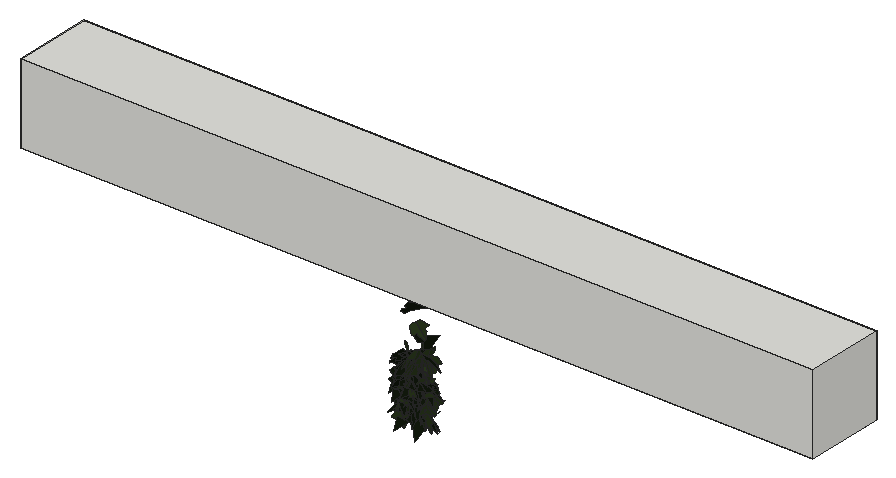
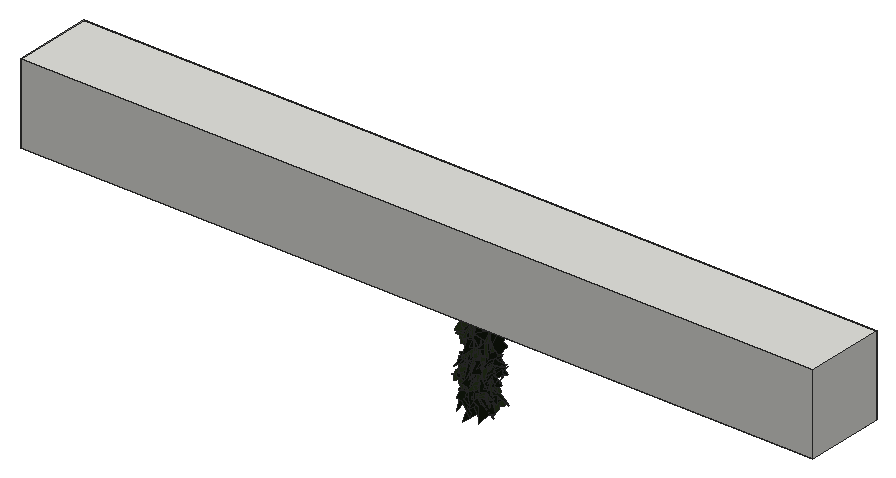
# SketchUp Ruby script. Lengths in inches.
U = 1.inch
M = Sketchup.active_model
def pt(a) = Geom::Point3d.new(a.map { |v| v * U })
def face(e, loops, mat)
  f = e.add_face(loops[0].map { |a| pt(a) })
  loops[1..].each { |l| e.add_face(l.map { |a| pt(a) }).erase! }
  f.material = f.back_material = mat if mat
  f
end
# faces: each face lists its corners as indices into pts; further lists are holes
def faces(e, pts, list, mat = nil) = list.each { |f| face(e, (f[0].is_a?(Array) ? f : [f]).map { |l| l.map { |i| pts[i] } }, mat) }
# xy, xz, yz: faces in a plane at the given z, y or x. An outline is a flat list of corners, or four numbers for a rectangle; further outlines are holes
def ring(l) = l.size == 4 ? [[l[0], l[1]], [l[2], l[1]], [l[2], l[3]], [l[0], l[3]]] : l.each_slice(2).to_a
def flat(e, list, mat, &to3) = list.each { |f| face(e, (f[0].is_a?(Array) ? f : [f]).map { |l| ring(l).map { |u, v| to3.(u, v) } }, mat) }
def xy(e, z, list, mat = nil) = flat(e, list, mat) { |x, y| [x, y, z] }
def xz(e, y, list, mat = nil) = flat(e, list, mat) { |x, z| [x, y, z] }
def yz(e, x, list, mat = nil) = flat(e, list, mat) { |y, z| [x, y, z] }
def lines(e, pts, list) = list.each { |a, b| e.add_line(pt(pts[a]), pt(pts[b])) }
# prism: a flat outline (further loops are holes) pulled along v
def prism(e, loops, v, mat = nil)
  f = face(e, loops, mat); d = Geom::Vector3d.new(v.map { |x| x * U })
  f.pushpull(f.normal.samedirection?(d) ? d.length : -d.length)
end
def box(e, o, s, mat = nil) = prism(e, [[o, [o[0] + s[0], o[1], o[2]], [o[0] + s[0], o[1] + s[1], o[2]], [o[0], o[1] + s[1], o[2]]]], [0, 0, s[2]], mat)
def at(x, y, z, deg = 0) = Geom::Transformation.translation(pt([x, y, z])) * Geom::Transformation.rotation(ORIGIN, Z_AXIS, deg.degrees)
def axes(o, x, y, z) = Geom::Transformation.new([*x, 0, *y, 0, *z, 0, *pt(o).to_a, 1])
def part(name) = M.definitions.add(name)
# library, detail: a bought-in or finely detailed component or shape, given as its bounding box
def library(name, o, s) = part(name).tap { |d| box(d.entities, o, s) }
def detail(e, o, s) = box(e.add_group.entities, o, s)
def put(e, d, t, mat = nil) = e.add_instance(d, t).tap { |i| i.material = mat if mat }
def group(e, t, mat = nil) = e.add_group.tap { |g| g.transformation = t; g.material = mat if mat }.entities
root = M.entities
M.materials.add("efeu1").color = [18, 25, 13]
M.materials.add("efeu2").color = [43, 57, 29]
c1 = part("ivyleaf_9")
p = [[1.54,2.16,1.25],[1.36,2.04,1.19],[-0.21,0.99,0.68],[-0.71,1.11,0.82],[-0.85,0.86,0.67],[-0.8,0.17,0.21],
  [-0.9,-0.01,0.1],[-0.67,-0.16,-0.02],[-0.08,-0.08,-0.05],[-0.03,-0.6,-0.4],[0.65,-0.88,-0.66],[0.83,-0.6,-0.49],
  [1.29,-0.42,-0.43],[1.8125,-0.07,-0.26],[1.21,0.44,0.15]]
faces(c1.entities,p,[[0,1,2,3,4,5,6,7,8,9,10,11,12,13,14]],"efeu1")
c2 = part("ivyleaf_10")
p = [[0,0.5,-0.03],[-0.0625,2.02,-0.43],[-0.19,2.01,-0.46],[-0.54,1.05,-0.29],[-0.52,0.625,-0.18],[-0.83,0.76,-0.28],
  [-1.16,0.64,-0.33],[-1.15,0.33,-0.24],[-0.77,-0.39,0.02],[-0.3,-0.51,0.16],[0.04,-0.48,0.23],[-0.02,2.01,-0.4375],
  [-0.06,2.01,-0.43],[0.04,-0.49,0.23],[0.67,-0.49,0.14],[1.38,0.36,-0.2],[1.375,0.51,-0.24],[0.81,0.65,-0.19],
  [0.62,0.59,-0.15],[0.6,1.09,-0.28],[0.5,1.23,-0.31]]
faces(c2.entities,p,[[0,1,2,3,4,5,6,7,8,9,10],[11,12,0,13,14,15,16,17,18,19,20]],"efeu2")
c3 = part("Agrupar\#1")
box(c3.entities,[0,0,0],[11.8125,11.8125,117.85])
put(root,c1,axes([28.08,223.79,225.72],[0.02886,0.49809,-0.03273],[-0.00222,-0.03265,-0.49893],[-0.49916,0.02895,0.00033]))
put(root,c1,axes([27.89,223.74,227.2],[0.24283,-0.01552,0.4368],[0.38825,0.23715,-0.20742],[-0.20073,0.43991,0.12722]))
put(root,c2,axes([29.64,223.99,223.66],[-0.44311,0.17665,-0.14984],[0.13435,-0.06751,-0.47686],[-0.1887,-0.46286,0.01236]))
put(root,c1,axes([28.35,224.14,226.5],[-0.11444,-0.44822,-0.18974],[0.05793,0.18099,-0.46248],[0.48327,-0.12783,0.0105]))
put(root,c1,axes([27.69,224.37,225.21],[-0.20659,-0.43058,0.14805],[-0.02291,-0.15254,-0.47561],[0.45475,-0.2033,0.0433]))
put(root,c2,axes([29.15,223.88,229.62],[0.38871,0.16806,0.26583],[0.18628,0.21748,-0.40988],[-0.25339,0.41768,0.10646]))
put(root,c2,axes([29.87,224.12,228.05],[-0.03679,-0.49505,0.05974],[-0.01741,-0.05859,-0.49625],[0.49834,-0.0386,-0.01293]))
put(root,c1,axes([27.66,223.7,226.98],[0.32776,0.14577,0.34831],[0.27906,0.21718,-0.35349],[-0.25435,0.42613,0.06101]))
put(root,c1,axes([29.08,224.26,225.62],[0.01884,-0.49961,-0.00573],[0.0001,0.00574,-0.49997],[0.49964,0.01884,0.00031]))
put(root,c2,axes([29.05,223.75,225.49],[0.11258,0.03787,-0.48569],[-0.25495,0.42935,-0.02562],[0.41512,0.25342,0.11599]))
put(root,c2,axes([29.4375,223.99,227.63],[-0.22597,0.44459,0.03575],[-0.11151,-0.01751,-0.48709],[-0.43186,-0.22811,0.10707]))
put(root,c2,axes([28.65,224.15,226.375],[0.01436,-0.49697,0.05308],[0.00715,-0.05289,-0.49714],[0.49974,0.01503,0.00559]))
put(root,c1,axes([28.82,224.37,225.66],[-0.40238,-0.27602,0.1091],[-0.05649,-0.10921,-0.48465],[0.29138,-0.40235,0.05671]))
put(root,c2,axes([29.37,223.95,228.08],[0.0604,-0.44788,-0.21391],[-0.01105,0.21422,-0.45165],[0.49621,0.05929,0.01598]))
put(root,c1,axes([29.62,224.07,227.94],[0.36342,-0.34323,-0.0108],[0.04273,0.06081,-0.49444],[0.34073,0.35846,0.07354]))
put(root,c2,axes([28.22,224.4,226.96],[-0.02444,-0.11259,0.48654],[0.29959,-0.39304,-0.07591],[0.39956,0.28782,0.08668]))
put(root,c1,axes([27.65,224.33,224.35],[0.08656,-0.47359,0.13496],[0.06393,-0.12507,-0.47987],[0.48828,0.10033,0.03891]))
put(root,c1,axes([29.05,224.14,225.96],[0.28799,-0.40729,-0.03437],[0.00679,0.0468,-0.49776],[0.40868,0.28623,0.03249]))
put(root,c1,axes([27.96,224.25,226.5],[-0.1452,0.25638,-0.40396],[0.18435,-0.35958,-0.29448],[-0.44151,-0.23446,0.00989]))
put(root,c2,axes([29.25,224.21,227.44],[0.14487,-0.46507,0.11279],[0.08301,-0.09163,-0.48447],[0.4713,0.15909,0.05067]))
put(root,c2,axes([27.95,224.05,223.21],[-0.428,-0.25848,-0.00276],[0.00172,0.00249,-0.49999],[0.25849,-0.428,-0.00124]))
put(root,c2,axes([29.11,224.14,227.64],[-0.1971,-0.45734,0.04464],[-0.01152,-0.04364,-0.49796],[0.45937,-0.19732,0.00666]))
put(root,c1,axes([29.04,224.34,225.98],[0.04844,-0.48903,0.09224],[-0.00287,-0.09295,-0.49128],[0.49764,0.04706,-0.01181]))
put(root,c1,axes([27.86,224.31,225.85],[-0.45881,-0.19855,-0.00827],[0.00771,0.00301,-0.49993],[0.19857,-0.45888,0.0003]))
put(root,c2,axes([28.69,224.18,226.7],[0.23462,-0.4398,0.03906],[0.04417,-0.02063,-0.49762],[0.43932,0.23696,0.02917]))
put(root,c2,axes([28.41,224.27,226.28],[0.04278,-0.47031,0.16425],[0.06965,-0.15759,-0.46938],[0.49327,0.06304,0.05203]))
put(root,c2,axes([29.97,224.38,225],[-0.01601,-0.37724,0.32777],[0.03658,-0.32794,-0.37565],[0.4984,0.01195,0.0381]))
put(root,c2,axes([28.31,224.16,226.29],[-0.3282,-0.37424,0.04724],[0.01601,-0.07638,-0.49387],[0.37687,-0.32266,0.06212]))
put(root,c2,axes([29.92,223.97,224.47],[-0.18144,-0.39912,-0.24037],[0.10621,0.21573,-0.43838],[0.45365,-0.21014,0.00649]))
put(root,c2,axes([27.97,224.4,227.36],[-0.04857,0.00726,0.49758],[0.40013,-0.29667,0.04338],[0.29586,0.40241,0.02301]))
put(root,c1,axes([28,224.2,224.09],[-0.41933,0.27097,-0.0271],[-0.02909,-0.09404,-0.49021],[-0.27077,-0.40955,0.09463]))
put(root,c2,axes([28.9,224.07,225.35],[0.13786,0.47909,0.03824],[-0.01892,0.04516,-0.4976],[-0.48025,0.13575,0.03058]))
put(root,c1,axes([28.99,224.41,224.59],[-0.09264,-0.49096,0.01946],[-0.0039,-0.01906,-0.49962],[0.49133,-0.09272,-0.0003]))
put(root,c1,axes([29.35,224.16,228.47],[-0.03235,-0.02391,0.49838],[0.45313,-0.21049,0.01931],[0.20888,0.45291,0.03528]))
put(root,c2,axes([29.01,224.22,226.66],[0.04699,-0.49764,0.0121],[-0.00477,-0.01261,-0.49982],[0.49776,0.04685,-0.00593]))
put(root,c1,axes([28.26,224.28,224.76],[0.192,-0.45988,-0.04052],[-0.00431,0.0421,-0.49821],[0.46165,0.19166,0.01221]))
put(root,c1,axes([29.65,224.42,225.6],[-0.35957,-0.3417,-0.06283],[0.0836,0.00267,-0.49295],[0.33722,-0.36501,0.05521]))
put(root,c2,axes([29.49,224.19,225.95],[-0.12805,-0.4833,-0.00529],[0.00747,0.00349,-0.49993],[0.48327,-0.12811,0.00633]))
put(root,c2,axes([28.42,224.125,226.28],[0.20173,-0.42766,-0.16251],[-0.07074,0.14631,-0.47285],[0.452,0.21377,-0.00148]))
put(root,c2,axes([29.4375,223.96,224.21],[-0.32826,0.21187,0.31202],[-0.25083,0.18627,-0.39037],[-0.28165,-0.41281,-0.016]))
put(root,c2,axes([28.59,224.23,226.64],[0.03796,-0.49851,-0.007],[-0.00081,0.00696,-0.49995],[0.49856,0.03797,-0.00028]))
put(root,c2,axes([29.24,224.29,224.65],[-0.19191,0.40614,-0.21959],[-0.00871,-0.24095,-0.43803],[-0.46162,-0.1643,0.09955]))
put(root,c2,axes([28.54,224.26,225.7],[0.10956,-0.48729,0.02331],[0.01029,-0.02157,-0.49943],[0.48774,0.10992,0.0053]))
put(root,c1,axes([28,224.54,223.18],[-0.32727,-0.35306,0.13507],[-0.01343,-0.16769,-0.47085],[0.37777,-0.31182,0.10028]))
put(root,c1,axes([28.63,224.34,224.07],[-0.36712,-0.08755,-0.32796],[0.32335,0.05681,-0.37712],[0.10329,-0.48899,0.01491]))
put(root,c2,axes([29.72,224.28,224.81],[-0.141,-0.47544,0.06382],[-0.00672,-0.06455,-0.49577],[0.47966,-0.14067,0.01181]))
put(root,c2,axes([29.81,224.1,227.17],[-0.18945,0.45842,0.06296],[-0.03302,0.05446,-0.49593],[-0.46154,-0.19206,0.00964]))
put(root,c2,axes([28.67,224.27,226.53],[0.06037,-0.49634,-0.0009],[0.0013,0.00106,-0.5],[0.49634,0.06036,0.00142]))
put(root,c1,axes([29,224.49,223.14],[-0.2094,-0.45398,0.00773],[-0.00021,-0.00842,-0.49993],[0.45404,-0.20937,0.00334]))
put(root,c1,axes([27.66,224.39,225.22],[0.09903,-0.48872,-0.03666],[-0.01438,0.03449,-0.4986],[0.48988,0.09981,-0.00722]))
put(root,c1,axes([27.84,224.26,225.05],[-0.16468,-0.09449,0.46255],[0.44317,-0.19981,0.11696],[0.16274,0.4485,0.14956]))
put(root,c2,axes([28.84,224.27,225.7],[-0.05793,-0.49663,-0.00036],[0.00152,0.00018,-0.5],[0.49663,-0.05793,0.00148]))
put(root,c1,axes([29.5,224.39,225.73],[0.10069,-0.4853,-0.06589],[0.00899,0.06909,-0.49512],[0.48967,0.09853,0.02264]))
put(root,c2,axes([29.29,224.33,224.96],[0.21042,-0.44519,0.08676],[0.15231,-0.02073,-0.47579],[0.42723,0.22666,0.12689]))
put(root,c2,axes([29.08,224.32,226.07],[-0.29824,-0.397,0.05867],[0.02576,-0.09189,-0.49081],[0.40048,-0.28974,0.07527]))
put(root,c1,axes([28.52,224.37,225.81],[0.47151,-0.01427,-0.16575],[0.1662,0.06224,0.46744],[0.00729,-0.49591,0.06343]))
put(root,c1,axes([29.34,224.14,226.41],[0.46793,-0.11445,-0.13396],[-0.12423,0.05528,-0.48116],[0.12494,0.48358,0.0233]))
put(root,c1,axes([28.22,224.375,225.73],[0.0332,-0.4728,-0.15924],[-0.0099,0.15894,-0.47396],[0.4988,0.03463,0.00119]))
put(root,c2,axes([29,224.43,223.73],[-0.00006,-0.47821,-0.14599],[0.02074,-0.14586,0.4778],[-0.49957,-0.00599,0.01985]))
put(root,c2,axes([28.125,224.3,226.32],[-0.22066,-0.44866,0.00342],[-0.00191,-0.00288,-0.49999],[0.44867,-0.22066,-0.00044]))
put(root,c1,axes([29.36,224.21,224.6],[-0.33714,0.36914,-0.00864],[0.00653,-0.00574,-0.49992],[-0.36918,-0.3372,-0.00096]))
put(root,c2,axes([28.07,224.2,224.25],[0.236,0.4389,0.04093],[-0.05509,0.07543,-0.4912],[-0.43734,0.22733,0.08396]))
put(root,c1,axes([28.92,224.4,224.63],[0.2176,-0.44969,-0.02073],[0.01216,0.02889,-0.49902],[0.45,0.21667,0.02351]))
put(root,c1,axes([28.73,224.1,227.48],[0.2293,0.39491,-0.20365],[-0.18554,-0.12313,-0.44768],[-0.40373,0.28087,0.09008]))
put(root,c2,axes([29.11,224.34,226.14],[0.47364,-0.15094,-0.05363],[-0.04977,0.02045,-0.4971],[0.15226,0.47623,0.00435]))
put(root,c1,axes([28.43,224.35,225.51],[-0.46934,0.17075,0.02376],[-0.02691,-0.00451,-0.49925],[-0.17028,-0.46992,0.01343]))
put(root,c2,axes([28.07,224.38,225.3],[-0.08507,-0.48901,0.06025],[-0.01642,-0.05829,-0.49632],[0.49244,-0.08643,-0.00614]))
put(root,c1,axes([28.4,223.92,230.58],[0.30254,0.30084,0.2607],[0.16311,0.20501,-0.42587],[-0.36313,0.34273,0.0259]))
put(root,c2,axes([29.89,224.25,227.51],[-0.48806,-0.10386,-0.03177],[0.0308,0.00789,-0.49899],[0.10415,-0.48903,-0.0013]))
put(root,c2,axes([29.49,224.29,224.34],[-0.40945,-0.28697,0.00173],[-0.00141,-0.001,-0.5],[0.28697,-0.40945,0.00001]))
put(root,c2,axes([29.45,224.34,225.16],[0.0538,-0.49568,-0.03756],[-0.00367,0.03738,-0.49859],[0.49708,0.05392,0.00038]))
put(root,c2,axes([28.54,224.34,226.43],[-0.36916,-0.32837,0.07677],[-0.05524,-0.0534,-0.49406],[0.33267,-0.37326,0.00315]))
put(root,c1,axes([29.59,224.22,225.64],[0.24221,0.31143,-0.30716],[-0.19927,-0.234,-0.39438],[-0.38939,0.31346,0.01076]))
put(root,c2,axes([29.47,224.28,225.07],[0.24079,0.43775,0.01989],[0.01183,0.0162,-0.4996],[-0.43804,0.24107,-0.00255]))
put(root,c2,axes([27.86,224.27,224.03],[-0.09051,-0.47369,-0.13201],[0.13118,0.1061,-0.47068],[0.47392,-0.11984,0.10507]))
put(root,c1,axes([29.48,224.24,225.77],[0.38304,-0.30792,-0.092],[0.02178,0.16769,-0.47054],[0.32063,0.35646,0.14188]))
put(root,c1,axes([28.61,224.21,227.1],[0.23252,0.35015,-0.27079],[-0.16585,-0.21468,-0.42001],[-0.4104,0.28514,0.01631]))
put(root,c2,axes([29.19,224.31,224.66],[0.30794,0.39389,0.00453],[0.00065,0.00524,-0.49997],[-0.39392,0.30793,0.00271]))
put(root,c1,axes([27.72,224.38,226.05],[0.14198,-0.45133,-0.16169],[0.0331,0.17746,-0.46628],[0.47827,0.1217,0.08027]))
put(root,c2,axes([28.31,224.24,226.77],[-0.47746,0.09288,0.11576],[-0.112,0.03041,-0.48634],[-0.09739,-0.49035,-0.00824]))
put(root,c2,axes([29.4,224.3,223.62],[-0.15562,0.47437,-0.02739],[-0.06755,-0.05062,-0.49282],[-0.47034,-0.14969,0.07985]))
put(root,c2,axes([28.59,224.39,224.84],[0.38534,-0.31533,0.04563],[0.07971,0.02608,-0.49292],[0.30848,0.38715,0.07037]))
put(root,c1,axes([28.71,224.23,225.52],[0.46354,-0.15223,-0.10934],[-0.09967,0.04683,-0.48772],[0.15873,0.47396,0.01307]))
put(root,c1,axes([29.06,224.08,227.16],[0.40132,0.29479,0.04517],[0.04282,0.01799,-0.49784],[-0.29514,0.40346,-0.01081]))
put(root,c1,axes([29.36,224.44,224.55],[-0.20905,-0.3247,-0.3176],[0.23865,0.21895,-0.38093],[0.38645,-0.31086,0.06343]))
put(root,c2,axes([28.61,224.41,224.42],[-0.13121,-0.48204,0.0206],[0.00604,-0.02299,-0.49943],[0.48244,-0.13081,0.01186]))
put(root,c1,axes([29.11,224.14,224.37],[0.26246,-0.00502,0.42555],[0.41387,0.11947,-0.25385],[-0.09913,0.48549,0.06687]))
put(root,c1,axes([29.04,224.31,224.96],[0.45974,-0.19271,-0.03876],[-0.03755,0.01066,-0.49847],[0.19295,0.46125,-0.00467]))
put(root,c2,axes([28.41,224.43,225.07],[-0.15538,-0.47441,0.02813],[-0.0044,-0.02816,-0.49919],[0.47522,-0.15538,0.00458]))
put(root,c1,axes([27.875,224.42,224.93],[0.35974,-0.34528,0.03692],[0.06591,0.01569,-0.49539],[0.34094,0.36129,0.0568]))
put(root,c2,axes([29.5,224.47,224.34],[-0.41931,-0.27234,0.00272],[0.078,-0.12487,-0.47783],[0.26094,-0.4003,0.1472]))
put(root,c2,axes([28.25,224.44,223.52],[0.47914,-0.04094,0.13694],[0.1387,0.01743,-0.48006],[0.03453,0.49802,0.02805]))
put(root,c2,axes([28.23,224.42,224.11],[0.23779,-0.43609,-0.0573],[0.00966,0.07031,-0.49494],[0.43973,0.23428,0.04187]))
put(root,c2,axes([29.33,224.2,227.03],[-0.08576,-0.05498,0.48951],[0.37205,0.31842,0.10094],[-0.32284,0.38156,-0.01371]))
put(root,c2,axes([29.4375,224.4,225.15],[-0.36871,-0.33771,-0.00129],[-0.00027,0.0022,-0.5],[0.33771,-0.36871,-0.00181]))
put(root,c1,axes([29.28,224.44,223.65],[0.3198,-0.38015,-0.05667],[0.00444,0.07737,-0.49396],[0.38432,0.31544,0.05287]))
put(root,c1,axes([28.87,224.5,224.38],[0.26949,-0.41934,-0.03907],[0.00971,0.05256,-0.49713],[0.42105,0.26719,0.03647]))
put(root,c1,axes([27.83,224.55,224.31],[-0.01026,-0.47767,-0.14741],[0.00806,0.14726,-0.47775],[0.49983,-0.01218,0.00468]))
put(root,c2,axes([28.08,224.43,226.79],[0.10485,-0.48354,-0.0721],[-0.00951,0.07171,-0.49474],[0.48879,0.10511,0.00584]))
put(root,c2,axes([28.42,224.25,225.76],[0.0817,-0.39276,-0.29844],[-0.00529,0.30179,-0.39861],[0.49325,0.0683,0.04516]))
put(root,c2,axes([29,224.58,223.83],[0.18279,-0.44119,0.14813],[0.13401,-0.1025,-0.47067],[0.44568,0.21177,0.08078]))
put(root,c2,axes([27.75,224.49,224.4375],[0.17655,-0.46688,-0.0292],[-0.00627,0.02885,-0.49913],[0.46775,0.17661,0.00434]))
put(root,c2,axes([29.48,224.2,225.58],[0.04746,0.40374,0.2911],[0.0373,0.28872,-0.40651],[-0.49634,0.06031,-0.00271]))
put(root,c2,axes([29.42,224.39,224.96],[0.29608,-0.34885,-0.2016],[-0.08857,0.18771,-0.45489],[0.39306,0.30507,0.04936]))
put(root,c2,axes([29.92,224.49,224.57],[-0.28118,-0.41344,0.00249],[-0.00643,0.00136,-0.49996],[0.4134,-0.28119,-0.00608]))
put(root,c1,axes([27.77,224.37,225.46],[0.42339,-0.26152,-0.04847],[0.05056,0.1686,-0.46799],[0.26113,0.39138,0.16921]))
put(root,c2,axes([29.21,224.41,223.66],[0.46141,-0.17771,-0.07431],[0.0001,0.19312,-0.4612],[0.19262,0.42559,0.17825]))
put(root,c1,axes([28.05,224.48,224.57],[-0.13875,0.45221,-0.16204],[0.01024,-0.16584,-0.47159],[-0.48026,-0.13418,0.03676]))
put(root,c2,axes([28.05,224.625,223.49],[0.3497,-0.35598,-0.03144],[-0.02278,0.0217,-0.49901],[0.35664,0.35044,-0.00104]))
put(root,c1,axes([29.4,224.26,225.6],[0.06829,-0.00685,-0.49527],[-0.39573,0.29991,-0.05871],[0.29788,0.40001,0.03554]))
put(root,c2,axes([28.83,224.52,224.27],[-0.47728,-0.14183,-0.04572],[0.04096,0.02264,-0.4978],[0.14328,-0.47893,-0.00999]))
put(root,c1,axes([28.57,224.35,223.5],[-0.05804,0.49579,0.02863],[-0.07054,0.02031,-0.49458],[-0.49158,-0.06145,0.06759]))
put(root,c1,axes([29.58,224.43,223.53],[0.45412,-0.02011,-0.20826],[-0.20604,0.04351,-0.45349],[0.03636,0.4977,0.03123]))
put(root,c1,axes([28.27,224.48,225.58],[0.08698,0.45825,-0.18012],[-0.02848,-0.17792,-0.46641],[-0.49155,0.0914,-0.00485]))
put(root,c2,axes([29.41,224.39,225.48],[-0.07287,0.1046,-0.48348],[-0.31091,0.37042,0.127],[0.38474,0.31914,0.01106]))
put(root,c2,axes([28.66,224.57,224.23],[0.03557,0.49525,0.05886],[-0.00025,0.05903,-0.4965],[-0.49873,0.03529,0.00444]))
put(root,c2,axes([27.79,224.37,223.82],[0.00631,-0.01626,0.4997],[0.17159,0.46945,0.01311],[-0.46959,0.17132,0.0115]))
put(root,c2,axes([29.13,224.625,223.35],[0.36433,-0.24005,-0.24421],[-0.15179,0.20642,-0.42936],[0.30696,0.38699,0.07753]))
put(root,c1,axes([28.33,224.4,223.92],[0.31426,0.3693,0.12187],[0.06747,0.10253,-0.4847],[-0.38299,0.32109,0.01461]))
put(root,c1,axes([28.46,224.68,223.43],[-0.38608,0.31547,0.03765],[-0.02757,0.02577,-0.49857],[-0.31651,-0.38706,-0.0025]))
put(root,c1,axes([28.91,224.48,223.43],[-0.01722,0.48181,0.13253],[-0.11042,0.12567,-0.47118],[-0.48735,-0.04549,0.10208]))
put(root,c1,axes([28.9,224.53,224.24],[0.14815,0.47459,0.05303],[-0.00454,0.05692,-0.49673],[-0.47753,0.1467,0.02117]))
put(root,c1,axes([29.45,224.6,223.15],[-0.00964,0.48609,0.11674],[-0.11918,0.11116,-0.47269],[-0.48549,-0.03694,0.11372]))
put(root,c1,axes([28.55,224.63,223.07],[0.39397,0.29653,0.08278],[0.06986,0.04482,-0.49306],[-0.29984,0.40007,-0.00611]))
put(root,c1,axes([27.95,224.68,223.24],[0.14406,0.4524,0.15678],[0.00192,0.16318,-0.47262],[-0.47879,0.13678,0.04528]))
put(root,c3,axes([58.92,223.4375,231.44],[0,0,0.5],[0,0.5,0],[-0.5,0,0]))
